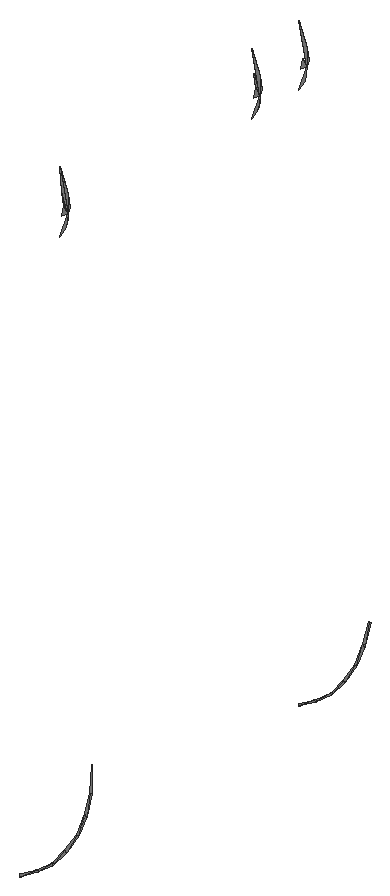
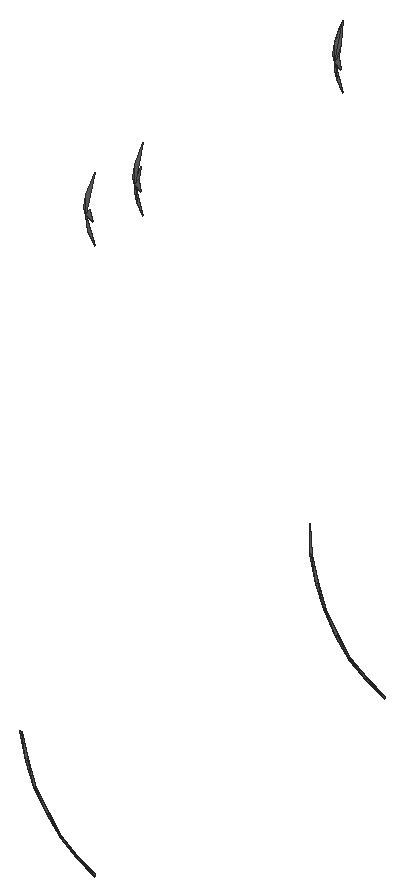
# SketchUp Ruby script. Lengths in inches.
U = 1.inch
M = Sketchup.active_model
def pt(a) = Geom::Point3d.new(a.map { |v| v * U })
def face(e, loops, mat)
  f = e.add_face(loops[0].map { |a| pt(a) })
  loops[1..].each { |l| e.add_face(l.map { |a| pt(a) }).erase! }
  f.material = f.back_material = mat if mat
  f
end
# faces: each face lists its corners as indices into pts; further lists are holes
def faces(e, pts, list, mat = nil) = list.each { |f| face(e, (f[0].is_a?(Array) ? f : [f]).map { |l| l.map { |i| pts[i] } }, mat) }
# xy, xz, yz: faces in a plane at the given z, y or x. An outline is a flat list of corners, or four numbers for a rectangle; further outlines are holes
def ring(l) = l.size == 4 ? [[l[0], l[1]], [l[2], l[1]], [l[2], l[3]], [l[0], l[3]]] : l.each_slice(2).to_a
def flat(e, list, mat, &to3) = list.each { |f| face(e, (f[0].is_a?(Array) ? f : [f]).map { |l| ring(l).map { |u, v| to3.(u, v) } }, mat) }
def xy(e, z, list, mat = nil) = flat(e, list, mat) { |x, y| [x, y, z] }
def xz(e, y, list, mat = nil) = flat(e, list, mat) { |x, z| [x, y, z] }
def yz(e, x, list, mat = nil) = flat(e, list, mat) { |y, z| [x, y, z] }
def lines(e, pts, list) = list.each { |a, b| e.add_line(pt(pts[a]), pt(pts[b])) }
# prism: a flat outline (further loops are holes) pulled along v
def prism(e, loops, v, mat = nil)
  f = face(e, loops, mat); d = Geom::Vector3d.new(v.map { |x| x * U })
  f.pushpull(f.normal.samedirection?(d) ? d.length : -d.length)
end
def box(e, o, s, mat = nil) = prism(e, [[o, [o[0] + s[0], o[1], o[2]], [o[0] + s[0], o[1] + s[1], o[2]], [o[0], o[1] + s[1], o[2]]]], [0, 0, s[2]], mat)
def at(x, y, z, deg = 0) = Geom::Transformation.translation(pt([x, y, z])) * Geom::Transformation.rotation(ORIGIN, Z_AXIS, deg.degrees)
def axes(o, x, y, z) = Geom::Transformation.new([*x, 0, *y, 0, *z, 0, *pt(o).to_a, 1])
def part(name) = M.definitions.add(name)
# library, detail: a bought-in or finely detailed component or shape, given as its bounding box
def library(name, o, s) = part(name).tap { |d| box(d.entities, o, s) }
def detail(e, o, s) = box(e.add_group.entities, o, s)
def put(e, d, t, mat = nil) = e.add_instance(d, t).tap { |i| i.material = mat if mat }
def group(e, t, mat = nil) = e.add_group.tap { |g| g.transformation = t; g.material = mat if mat }.entities
root = M.entities
M.materials.add("Material \#1").color = [140, 140, 140]
xz(root,115.85,[[101.59,190.81,101.59,190.82,101.68,190.87],[101.59,190.81,101.68,190.87,101.68,190.86],[101.68,190.86,101.68,190.87,101.76,190.93],[101.68,190.86,101.76,190.93,101.76,190.92],[101.76,190.92,101.76,190.93,101.82,191.01],
  [101.76,190.92,101.82,191.01,101.83,191],[101.83,191,101.82,191.01,101.88,191.1],[101.83,191,101.88,191.1,101.89,191.1],[101.88,191.1,101.92,191.21,101.89,191.1],[101.89,191.1,101.92,191.21,101.93,191.2],
  [101.93,191.2,101.92,191.21,101.95,191.32],[101.93,191.2,101.95,191.32,101.96,191.32],[101.95,191.32,101.96,191.45,101.96,191.32]],"Material \#1")
xz(root,116.13,[[101.57,193.61,101.6,193.66,101.61,193.73],[101.6,193.66,101.61,193.7,101.61,193.73],[101.58,193.71,101.61,193.73,101.59,193.76],[101.61,193.73,101.57,193.93,101.58,193.82],[101.61,193.73,101.61,193.82,101.57,193.93],
  [101.61,193.73,101.58,193.82,101.59,193.76],[101.61,193.73,101.62,193.76,101.61,193.82],[101.61,193.82,101.59,193.88,101.57,193.93]],"Material \#1")
xz(root,117.36,[[101.57,193.61,101.61,193.73,101.6,193.66],[101.6,193.66,101.61,193.73,101.61,193.7],[101.58,193.71,101.59,193.76,101.61,193.73],[101.61,193.73,101.57,193.93,101.61,193.82],[101.61,193.73,101.59,193.76,101.58,193.82],
  [101.61,193.73,101.61,193.82,101.62,193.76]],"Material \#1")
xz(root,117.63,[[101.59,190.81,101.68,190.86,101.68,190.87],[101.59,190.81,101.68,190.87,101.59,190.82],[101.68,190.86,101.76,190.92,101.76,190.93],[101.68,190.86,101.76,190.93,101.68,190.87],[101.76,190.92,101.82,191.01,101.76,190.93],
  [101.76,190.92,101.83,191,101.82,191.01],[101.83,191,101.88,191.1,101.82,191.01],[101.83,191,101.89,191.1,101.88,191.1],[101.88,191.1,101.89,191.1,101.92,191.21],[101.89,191.1,101.93,191.2,101.92,191.21],
  [101.93,191.2,101.95,191.32,101.92,191.21],[101.93,191.2,101.96,191.32,101.95,191.32]],"Material \#1")
xz(root,117.66,[[101.57,193.61,101.6,193.66,101.61,193.73],[101.58,193.71,101.61,193.73,101.59,193.76],[101.61,193.73,101.61,193.82,101.57,193.93],[101.61,193.73,101.62,193.76,101.61,193.82]],"Material \#1")
